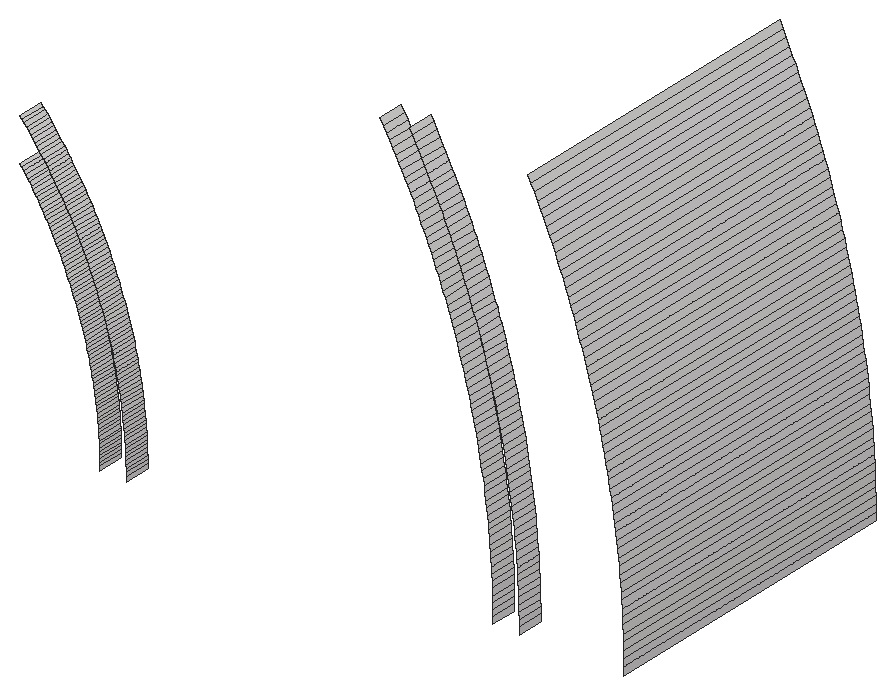
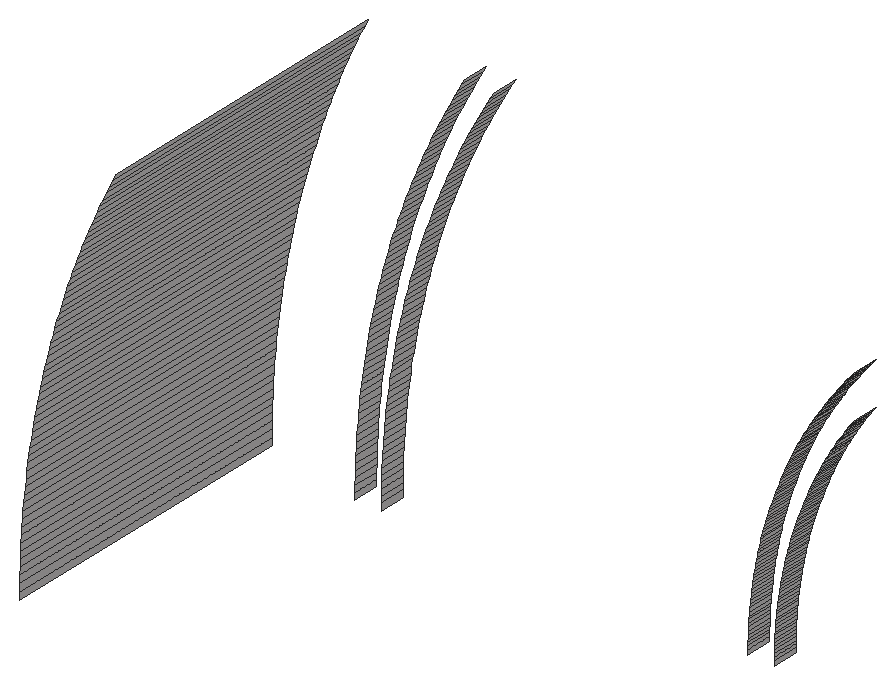
# SketchUp Ruby script. Lengths in inches.
U = 1.inch
M = Sketchup.active_model
def pt(a) = Geom::Point3d.new(a.map { |v| v * U })
def face(e, loops, mat)
  f = e.add_face(loops[0].map { |a| pt(a) })
  loops[1..].each { |l| e.add_face(l.map { |a| pt(a) }).erase! }
  f.material = f.back_material = mat if mat
  f
end
# faces: each face lists its corners as indices into pts; further lists are holes
def faces(e, pts, list, mat = nil) = list.each { |f| face(e, (f[0].is_a?(Array) ? f : [f]).map { |l| l.map { |i| pts[i] } }, mat) }
# xy, xz, yz: faces in a plane at the given z, y or x. An outline is a flat list of corners, or four numbers for a rectangle; further outlines are holes
def ring(l) = l.size == 4 ? [[l[0], l[1]], [l[2], l[1]], [l[2], l[3]], [l[0], l[3]]] : l.each_slice(2).to_a
def flat(e, list, mat, &to3) = list.each { |f| face(e, (f[0].is_a?(Array) ? f : [f]).map { |l| ring(l).map { |u, v| to3.(u, v) } }, mat) }
def xy(e, z, list, mat = nil) = flat(e, list, mat) { |x, y| [x, y, z] }
def xz(e, y, list, mat = nil) = flat(e, list, mat) { |x, z| [x, y, z] }
def yz(e, x, list, mat = nil) = flat(e, list, mat) { |y, z| [x, y, z] }
def lines(e, pts, list) = list.each { |a, b| e.add_line(pt(pts[a]), pt(pts[b])) }
# prism: a flat outline (further loops are holes) pulled along v
def prism(e, loops, v, mat = nil)
  f = face(e, loops, mat); d = Geom::Vector3d.new(v.map { |x| x * U })
  f.pushpull(f.normal.samedirection?(d) ? d.length : -d.length)
end
def box(e, o, s, mat = nil) = prism(e, [[o, [o[0] + s[0], o[1], o[2]], [o[0] + s[0], o[1] + s[1], o[2]], [o[0], o[1] + s[1], o[2]]]], [0, 0, s[2]], mat)
def at(x, y, z, deg = 0) = Geom::Transformation.translation(pt([x, y, z])) * Geom::Transformation.rotation(ORIGIN, Z_AXIS, deg.degrees)
def axes(o, x, y, z) = Geom::Transformation.new([*x, 0, *y, 0, *z, 0, *pt(o).to_a, 1])
def part(name) = M.definitions.add(name)
# library, detail: a bought-in or finely detailed component or shape, given as its bounding box
def library(name, o, s) = part(name).tap { |d| box(d.entities, o, s) }
def detail(e, o, s) = box(e.add_group.entities, o, s)
def put(e, d, t, mat = nil) = e.add_instance(d, t).tap { |i| i.material = mat if mat }
def group(e, t, mat = nil) = e.add_group.tap { |g| g.transformation = t; g.material = mat if mat }.entities
root = M.entities
M.materials.add("[Quartz Light Brown]").color = [215, 212, 212]
yz(root,519.98,[[38,84.75,39,84.88]],"[Quartz Light Brown]")
yz(root,519.99,[[38,84.5,39,84.63]],"[Quartz Light Brown]")
yz(root,520,[[38,83.96,39,84.125],[38,84.125,39,84.25],[38,84.25,39,84.375]],"[Quartz Light Brown]")
yz(root,520.97,[[38,84.93,39,85.07]],"[Quartz Light Brown]")
yz(root,520.99,[[38,84.53,39,84.67]],"[Quartz Light Brown]")
yz(root,521,[[38,83.96,39,84.13],[38,84.13,39,84.27],[38,84.27,39,84.4]],"[Quartz Light Brown]")
yz(root,534.98,[[38,84.97,39,85.22]],"[Quartz Light Brown]")
yz(root,535,[[38,83.99,39,84.24],[38,84.24,39,84.49]],"[Quartz Light Brown]")
yz(root,535.98,[[38,85.01,39,85.26]],"[Quartz Light Brown]")
yz(root,536,[[38,83.99,39,84.25],[38,84.25,39,84.5]],"[Quartz Light Brown]")
yz(root,540,[[38,84,50,84.28],[38,84.28,50,84.57]],"[Quartz Light Brown]")
p = [[519.99,39,84.5],[519.99,38,84.5],[520,38,84.375],[520,39,84.375],[520.99,38,84.53],[520.99,39,84.53],
  [521,39,84.4],[521,38,84.4],[534.99,39,84.73],[534.99,38,84.73],[535,38,84.49],[535,39,84.49],
  [535.99,38,84.75],[535.99,39,84.75],[536,39,84.5],[536,38,84.5],[519.98,39,84.75],[519.98,38,84.75],
  [519.99,38,84.63],[519.99,39,84.63],[539.99,38,84.85],[540,38,84.57],[540,50,84.57],[539.99,50,84.85],
  [520.98,38,84.8],[520.98,39,84.8],[520.99,39,84.67],[520.99,38,84.67],[534.98,39,84.97],[534.98,38,84.97],
  [520.97,38,84.93],[520.97,39,84.93],[535.98,38,85.01],[535.98,39,85.01],[539.98,38,85.13],[539.98,50,85.13],
  [519.97,39,85],[519.97,38,85],[519.98,38,84.88],[519.98,39,84.88],[519.96,39,85.13],[519.96,38,85.13],
  [519.95,39,85.26],[519.95,38,85.26],[520.96,38,85.2],[520.96,39,85.2],[520.97,39,85.07],[520.97,38,85.07],
  [539.97,38,85.41],[539.97,50,85.41],[520.95,38,85.33],[520.95,39,85.33],[534.97,39,85.46],[534.97,38,85.46],
  [534.98,38,85.22],[534.98,39,85.22],[519.94,39,85.38],[519.94,38,85.38],[520.9375,38,85.47],[520.9375,39,85.47],
  [535.96,38,85.51],[535.96,39,85.51],[535.98,39,85.26],[535.98,38,85.26],[519.93,39,85.51],[519.93,38,85.51],
  [539.96,38,85.7],[539.96,50,85.7],[519.92,39,85.63],[519.92,38,85.63],[520.92,38,85.6],[520.92,39,85.6],
  [534.95,39,85.7],[534.95,38,85.7],[535.95,38,85.76],[535.95,39,85.76],[519.9,39,85.76],[519.9,38,85.76],
  [520.91,38,85.73],[520.91,39,85.73],[520.9,38,85.87],[520.9,39,85.87],[534.9375,39,85.95],[534.9375,38,85.95],
  [539.95,38,85.98],[539.95,50,85.98],[519.89,39,85.88],[519.89,38,85.88],[535.9375,38,86.01],[535.9375,39,86.01],
  [519.875,39,86.01],[519.875,38,86.01],[520.88,38,86],[520.88,39,86],[534.92,39,86.1875],[534.92,38,86.1875],
  [519.86,39,86.13],[519.86,38,86.13],[520.87,38,86.13],[520.87,39,86.13],[535.92,38,86.26],[535.92,39,86.26],
  [539.93,38,86.26],[539.93,50,86.26],[519.84,39,86.25],[519.84,38,86.25],[520.85,38,86.26],[520.85,39,86.26],
  [534.9,39,86.43],[534.9,38,86.43],[519.82,39,86.38],[519.82,38,86.38],[520.83,38,86.4],[520.83,39,86.4],
  [535.9,38,86.51],[535.9,39,86.51],[539.91,38,86.54],[539.91,50,86.54],[519.8,39,86.5],[519.8,38,86.5],
  [520.8125,38,86.53],[520.8125,39,86.53],[534.88,39,86.67],[534.88,38,86.67],[519.78,39,86.625],[519.78,38,86.625],
  [520.79,38,86.66],[520.79,39,86.66],[535.88,38,86.76],[535.88,39,86.76],[539.89,38,86.82],[539.89,50,86.82],
  [519.76,39,86.75],[519.76,38,86.75],[520.77,38,86.79],[520.77,39,86.79],[534.86,39,86.92],[534.86,38,86.92],
  [519.74,39,86.875],[519.74,38,86.875],[520.75,38,86.92],[520.75,39,86.92],[535.86,38,87.01],[535.86,39,87.01],
  [539.87,38,87.11],[539.87,50,87.11],[519.72,39,87],[519.72,38,87],[520.72,38,87.05],[520.72,39,87.05],
  [534.84,39,87.16],[534.84,38,87.16],[519.69,39,87.12],[519.69,38,87.12],[535.83,38,87.26],[535.83,39,87.26],
  [519.67,39,87.24],[519.67,38,87.24],[520.7,38,87.19],[520.7,39,87.19],[539.84,38,87.39],[539.84,50,87.39],
  [519.64,39,87.37],[519.64,38,87.37],[520.67,38,87.32],[520.67,39,87.32],[534.8125,39,87.4],[534.8125,38,87.4],
  [520.65,38,87.45],[520.65,39,87.45],[535.81,38,87.51],[535.81,39,87.51],[519.61,39,87.49],[519.61,38,87.49],
  [520.62,38,87.58],[520.62,39,87.58],[534.79,39,87.64],[534.79,38,87.64],[539.8125,38,87.67],[539.8125,50,87.67],
  [519.59,39,87.61],[519.59,38,87.61],[535.78,38,87.76],[535.78,39,87.76],[519.56,39,87.74],[519.56,38,87.74],
  [520.59,38,87.71],[520.59,39,87.71],[534.76,39,87.89],[534.76,38,87.89],[519.53,39,87.86],[519.53,38,87.86],
  [520.5625,38,87.84],[520.5625,39,87.84],[539.78,38,87.95],[539.78,50,87.95],[520.53,38,87.97],[520.53,39,87.97],
  [535.75,38,88.01],[535.75,39,88.01],[519.5,39,87.98],[519.5,38,87.98],[534.72,39,88.125],[534.72,38,88.125],
  [519.47,39,88.1],[519.47,38,88.1],[520.5,38,88.1],[520.5,39,88.1],[535.72,38,88.26],[535.72,39,88.26],
  [539.75,38,88.23],[539.75,50,88.23],[519.43,39,88.22],[519.43,38,88.22],[520.47,38,88.23],[520.47,39,88.23],
  [534.69,39,88.37],[534.69,38,88.37],[519.4,39,88.34],[519.4,38,88.34],[520.43,38,88.36],[520.43,39,88.36],
  [539.72,38,88.51],[539.72,50,88.51],[519.36,39,88.46],[519.36,38,88.46],[535.68,38,88.51],[535.68,39,88.51],
  [520.4,38,88.49],[520.4,39,88.49],[534.66,39,88.61],[534.66,38,88.61],[519.33,39,88.58],[519.33,38,88.58],
  [520.36,38,88.61],[520.36,39,88.61],[535.64,38,88.76],[535.64,39,88.76],[539.68,38,88.79],[539.68,50,88.79],
  [519.29,39,88.7],[519.29,38,88.7],[520.32,38,88.74],[520.32,39,88.74],[534.62,39,88.85],[534.62,38,88.85],
  [519.26,39,88.82],[519.26,38,88.82],[520.29,38,88.87],[520.29,39,88.87],[519.22,39,88.94],[519.22,38,88.94],
  [534.58,39,89.09],[534.58,38,89.09],[535.61,38,89.01],[535.61,39,89.01],[539.64,38,89.07],[539.64,50,89.07],
  [519.18,39,89.0625],[519.18,38,89.0625],[520.25,38,89],[520.25,39,89],[520.21,38,89.125],[520.21,39,89.125],
  [535.57,38,89.25],[535.57,39,89.25],[519.14,39,89.18],[519.14,38,89.18],[520.17,38,89.25],[520.17,39,89.25],
  [534.54,39,89.33],[534.54,38,89.33],[539.6,38,89.35],[539.6,50,89.35],[519.1,39,89.3],[519.1,38,89.3],
  [519.05,39,89.42],[519.05,38,89.42],[520.125,38,89.38],[520.125,39,89.38],[534.5,39,89.57],[534.5,38,89.57],
  [535.52,38,89.5],[535.52,39,89.5],[519.01,39,89.54],[519.01,38,89.54],[520.08,38,89.51],[520.08,39,89.51],
  [539.56,38,89.63],[539.56,50,89.63],[518.97,39,89.66],[518.97,38,89.66],[520.04,38,89.63],[520.04,39,89.63],
  [535.48,38,89.75],[535.48,39,89.75],[519.99,38,89.76],[519.99,39,89.76],[534.45,39,89.81],[534.45,38,89.81],
  [539.51,38,89.91],[539.51,50,89.91],[518.92,39,89.77],[518.92,38,89.77],[535.43,38,90],[535.43,39,90],
  [518.875,39,89.89],[518.875,38,89.89],[519.95,38,89.88],[519.95,39,89.88],[534.4,39,90.05],[534.4,38,90.05],
  [518.83,39,90.01],[518.83,38,90.01],[519.9,38,90.01],[519.9,39,90.01],[539.46,38,90.1875],[539.46,50,90.1875],
  [518.78,39,90.12],[518.78,38,90.12],[519.85,38,90.13],[519.85,39,90.13],[534.36,39,90.29],[534.36,38,90.29],
  [535.39,38,90.24],[535.39,39,90.24],[518.73,39,90.24],[518.73,38,90.24],[519.81,38,90.26],[519.81,39,90.26],
  [518.68,39,90.35],[518.68,38,90.35],[535.34,38,90.49],[535.34,39,90.49],[539.41,38,90.47],[539.41,50,90.47],
  [519.76,38,90.38],[519.76,39,90.38],[534.31,39,90.52],[534.31,38,90.52],[518.63,39,90.47],[518.63,38,90.47],
  [519.71,38,90.51],[519.71,39,90.51],[518.58,39,90.58],[518.58,38,90.58],[519.65,38,90.63],[519.65,39,90.63],
  [534.25,39,90.76],[534.25,38,90.76],[535.28,38,90.74],[535.28,39,90.74],[539.36,38,90.75],[539.36,50,90.75],
  [518.53,39,90.7],[518.53,38,90.7],[519.6,38,90.75],[519.6,39,90.75],[518.48,39,90.8125],[518.48,38,90.8125],
  [535.23,38,90.98],[535.23,39,90.98],[539.31,38,91.02],[539.31,50,91.02],[518.42,39,90.93],[518.42,38,90.93],
  [519.55,38,90.875],[519.55,39,90.875],[534.2,39,91],[534.2,38,91],[518.37,39,91.04],[518.37,38,91.04],
  [519.49,38,91],[519.49,39,91],[518.3125,39,91.15],[518.3125,38,91.15],[519.4375,38,91.12],[519.4375,39,91.12],
  [534.14,39,91.24],[534.14,38,91.24],[535.17,38,91.23],[535.17,39,91.23],[539.25,38,91.3],[539.25,50,91.3],
  [519.38,38,91.24],[519.38,39,91.24],[518.26,39,91.26],[518.26,38,91.26],[519.32,38,91.36],[519.32,39,91.36],
  [534.09,39,91.47],[534.09,38,91.47],[535.12,38,91.47],[535.12,39,91.47],[518.2,39,91.375],[518.2,38,91.375],
  [539.19,38,91.58],[539.19,50,91.58],[518.14,39,91.49],[518.14,38,91.49],[519.27,38,91.48],[519.27,39,91.48],
  [518.08,39,91.6],[518.08,38,91.6],[519.21,38,91.6],[519.21,39,91.6],[534.03,39,91.71],[534.03,38,91.71],
  [535.06,38,91.71],[535.06,39,91.71],[518.02,39,91.71],[518.02,38,91.71],[519.15,38,91.72],[519.15,39,91.72],
  [539.13,38,91.85],[539.13,50,91.85],[517.96,39,91.82],[517.96,38,91.82],[519.09,38,91.84],[519.09,39,91.84],
  [533.96,39,91.94],[533.96,38,91.94],[534.99,38,91.96],[534.99,39,91.96],[517.9,39,91.93],[517.9,38,91.93],
  [519.02,38,91.95],[519.02,39,91.95],[517.84,39,92.04],[517.84,38,92.04],[533.9,39,92.18],[533.9,38,92.18],
  [539.07,38,92.13],[539.07,50,92.13],[517.77,39,92.14],[517.77,38,92.14],[518.96,38,92.07],[518.96,39,92.07],
  [534.93,38,92.2],[534.93,39,92.2],[517.71,39,92.25],[517.71,38,92.25],[518.9,38,92.19],[518.9,39,92.19],
  [539.01,38,92.4],[539.01,50,92.4],[518.83,38,92.31],[518.83,39,92.31],[533.84,39,92.41],[533.84,38,92.41],
  [534.87,38,92.44],[534.87,39,92.44],[517.64,39,92.36],[517.64,38,92.36],[518.77,38,92.42],[518.77,39,92.42],
  [517.58,39,92.47],[517.58,38,92.47],[518.7,38,92.54],[518.7,39,92.54],[533.77,39,92.65],[533.77,38,92.65],
  [534.8,38,92.6875],[534.8,39,92.6875],[538.9375,38,92.68],[538.9375,50,92.68],[517.51,39,92.57],[517.51,38,92.57],
  [518.63,38,92.65],[518.63,39,92.65],[517.44,39,92.68],[517.44,38,92.68],[533.7,39,92.88],[533.7,38,92.88],
  [517.37,39,92.78],[517.37,38,92.78],[518.5625,38,92.77],[518.5625,39,92.77],[534.73,38,92.93],[534.73,39,92.93],
  [538.87,38,92.95],[538.87,50,92.95],[517.3,39,92.89],[517.3,38,92.89],[518.49,38,92.88],[518.49,39,92.88],
  [517.23,39,92.99],[517.23,38,92.99],[518.42,38,93],[518.42,39,93],[533.63,39,93.12],[533.63,38,93.12],
  [534.66,38,93.17],[534.66,39,93.17],[517.16,39,93.1],[517.16,38,93.1],[518.35,38,93.11],[518.35,39,93.11],
  [538.8,38,93.23],[538.8,50,93.23],[517.09,39,93.2],[517.09,38,93.2],[518.28,38,93.22],[518.28,39,93.22],
  [533.56,39,93.35],[533.56,38,93.35],[517.02,39,93.3],[517.02,38,93.3],[518.21,38,93.33],[518.21,39,93.33],
  [534.59,38,93.41],[534.59,39,93.41],[538.72,38,93.5],[538.72,50,93.5],[516.94,39,93.4],[516.94,38,93.4],
  [518.13,38,93.44],[518.13,39,93.44],[533.48,39,93.58],[533.48,38,93.58],[518.06,38,93.56],[518.06,39,93.56],
  [534.51,38,93.65],[534.51,39,93.65],[538.65,38,93.77],[538.65,50,93.77],[517.98,38,93.67],[517.98,39,93.67],
  [533.41,39,93.8125],[533.41,38,93.8125],[534.43,38,93.89],[534.43,39,93.89],[517.91,38,93.78],[517.91,39,93.78],
  [517.83,38,93.88],[517.83,39,93.88],[533.33,39,94.04],[533.33,38,94.04],[538.57,38,94.04],[538.57,50,94.04],
  [517.75,38,93.99],[517.75,39,93.99],[534.36,38,94.13],[534.36,39,94.13],[517.67,38,94.1],[517.67,39,94.1],
  [533.25,39,94.27],[533.25,38,94.27],[538.49,38,94.31],[538.49,50,94.31],[517.59,38,94.21],[517.59,39,94.21],
  [534.27,38,94.37],[534.27,39,94.37],[517.51,38,94.3125],[517.51,39,94.3125],[517.43,38,94.42],[517.43,39,94.42],
  [533.17,39,94.5],[533.17,38,94.5],[538.41,38,94.59],[538.41,50,94.59],[517.35,38,94.52],[517.35,39,94.52],
  [534.19,38,94.6],[534.19,39,94.6],[517.27,38,94.63],[517.27,39,94.63],[533.08,39,94.73],[533.08,38,94.73],
  [517.18,38,94.73],[517.18,39,94.73],[534.11,38,94.84],[534.11,39,94.84],[538.32,38,94.86],[538.32,50,94.86],
  [517.1,38,94.84],[517.1,39,94.84],[533,39,94.96],[533,38,94.96],[517.01,38,94.9375],[517.01,39,94.9375],
  [534.02,38,95.08],[534.02,39,95.08],[516.93,38,95.04],[516.93,39,95.04],[538.24,38,95.125],[538.24,50,95.125],
  [532.91,39,95.19],[532.91,38,95.19],[533.93,38,95.3125],[533.93,39,95.3125],[538.15,38,95.39],[538.15,50,95.39],
  [532.82,39,95.41],[532.82,38,95.41],[533.84,38,95.55],[533.84,39,95.55],[532.73,39,95.64],[532.73,38,95.64],
  [538.06,38,95.66],[538.06,50,95.66],[533.75,38,95.78],[533.75,39,95.78],[532.64,39,95.86],[532.64,38,95.86],
  [537.97,38,95.93],[537.97,50,95.93],[533.66,38,96.01],[533.66,39,96.01],[532.55,39,96.09],[532.55,38,96.09],
  [537.87,38,96.19],[537.87,50,96.19],[533.5625,38,96.25],[533.5625,39,96.25],[532.45,39,96.3125],[532.45,38,96.3125],
  [533.47,38,96.48],[533.47,39,96.48],[537.77,38,96.46],[537.77,50,96.46],[532.35,39,96.53],[532.35,38,96.53],
  [532.25,39,96.76],[532.25,38,96.76],[533.37,38,96.71],[533.37,39,96.71],[537.68,38,96.73],[537.68,50,96.73],
  [533.27,38,96.9375],[533.27,39,96.9375],[537.58,38,96.99],[537.58,50,96.99],[532.15,39,96.98],[532.15,38,96.98],
  [533.16,38,97.17],[533.16,39,97.17],[532.05,39,97.2],[532.05,38,97.2],[537.47,38,97.25],[537.47,50,97.25],
  [531.95,39,97.42],[531.95,38,97.42],[533.0625,38,97.4],[533.0625,39,97.4],[537.37,38,97.51],[537.37,50,97.51],
  [531.84,39,97.64],[531.84,38,97.64],[532.95,38,97.625],[532.95,39,97.625],[537.26,38,97.78],[537.26,50,97.78],
  [531.73,39,97.86],[531.73,38,97.86],[532.85,38,97.85],[532.85,39,97.85],[537.15,38,98.04],[537.15,50,98.04],
  [531.62,39,98.07],[531.62,38,98.07],[532.74,38,98.08],[532.74,39,98.08],[537.04,38,98.3],[537.04,50,98.3],
  [531.51,39,98.29],[531.51,38,98.29],[532.625,38,98.3],[532.625,39,98.3],[531.4,39,98.51],[531.4,38,98.51],
  [532.51,38,98.53],[532.51,39,98.53],[536.93,38,98.56],[536.93,50,98.56],[531.28,39,98.72],[531.28,38,98.72],
  [532.4,38,98.75],[532.4,39,98.75],[536.8125,38,98.81],[536.8125,50,98.81],[531.17,39,98.93],[531.17,38,98.93],
  [532.28,38,98.97],[532.28,39,98.97],[536.69,38,99.07],[536.69,50,99.07],[531.05,39,99.15],[531.05,38,99.15],
  [532.16,38,99.2],[532.16,39,99.2],[530.93,39,99.36],[530.93,38,99.36],[536.57,38,99.33],[536.57,50,99.33],
  [532.04,38,99.42],[532.04,39,99.42],[536.45,38,99.58],[536.45,50,99.58],[530.81,39,99.57],[530.81,38,99.57],
  [531.92,38,99.64],[531.92,39,99.64],[530.68,39,99.78],[530.68,38,99.78],[531.8,38,99.85],[531.8,39,99.85],
  [536.33,38,99.84],[536.33,50,99.84]]
faces(root,p,[[0,1,2,3],[4,5,6,7],[8,9,10,11],[12,13,14,15],[16,17,18,19],[20,21,22,23],[24,25,26,27],[28,29,9,8],
  [30,31,25,24],[32,33,13,12],[34,20,23,35],[36,37,38,39],[40,41,37,36],[42,43,41,40],[44,45,46,47],[48,34,35,49],
  [50,51,45,44],[52,53,54,55],[56,57,43,42],[58,59,51,50],[60,61,62,63],[64,65,57,56],[66,48,49,67],[68,69,65,64],
  [70,71,59,58],[72,73,53,52],[74,75,61,60],[76,77,69,68],[78,79,71,70],[80,81,79,78],[82,83,73,72],[84,66,67,85],
  [86,87,77,76],[88,89,75,74],[90,91,87,86],[92,93,81,80],[94,95,83,82],[96,97,91,90],[98,99,93,92],[100,101,89,88],
  [102,84,85,103],[104,105,97,96],[106,107,99,98],[108,109,95,94],[110,111,105,104],[112,113,107,106],[114,115,101,100],[116,102,103,117],
  [118,119,111,110],[120,121,113,112],[122,123,109,108],[124,125,119,118],[126,127,121,120],[128,129,115,114],[130,116,117,131],[132,133,125,124],
  [134,135,127,126],[136,137,123,122],[138,139,133,132],[140,141,135,134],[142,143,129,128],[144,130,131,145],[146,147,139,138],[148,149,141,140],
  [150,151,137,136],[152,153,147,146],[154,155,143,142],[156,157,153,152],[158,159,149,148],[160,144,145,161],[162,163,157,156],[164,165,159,158],
  [166,167,151,150],[168,169,165,164],[170,171,155,154],[172,173,163,162],[174,175,169,168],[176,177,167,166],[178,160,161,179],[180,181,173,172],
  [182,183,171,170],[184,185,181,180],[186,187,175,174],[188,189,177,176],[190,191,185,184],[192,193,187,186],[194,178,179,195],[196,197,193,192],
  [198,199,183,182],[200,201,191,190],[202,203,189,188],[204,205,201,200],[206,207,197,196],[208,209,199,198],[210,194,195,211],[212,213,205,204],
  [214,215,207,206],[216,217,203,202],[218,219,213,212],[220,221,215,214],[222,210,211,223],[224,225,219,218],[226,227,209,208],[228,229,221,220],
  [230,231,217,216],[232,233,225,224],[234,235,229,228],[236,237,227,226],[238,222,223,239],[240,241,233,232],[242,243,235,234],[244,245,231,230],
  [246,247,241,240],[248,249,243,242],[250,251,247,246],[252,253,245,244],[254,255,237,236],[256,238,239,257],[258,259,251,250],[260,261,249,248],
  [262,263,261,260],[264,265,255,254],[266,267,259,258],[268,269,263,262],[270,271,253,252],[272,256,257,273],[274,275,267,266],[276,277,275,274],
  [278,279,269,268],[280,281,271,270],[282,283,265,264],[284,285,277,276],[286,287,279,278],[288,272,273,289],[290,291,285,284],[292,293,287,286],
  [294,295,283,282],[296,297,293,292],[298,299,281,280],[300,288,289,301],[302,303,291,290],[304,305,295,294],[306,307,303,302],[308,309,297,296],
  [310,311,299,298],[312,313,307,306],[314,315,309,308],[316,300,301,317],[318,319,313,312],[320,321,315,314],[322,323,311,310],[324,325,305,304],
  [326,327,319,318],[328,329,321,320],[330,331,327,326],[332,333,325,324],[334,316,317,335],[336,337,329,328],[338,339,323,322],[340,341,331,330],
  [342,343,337,336],[344,345,341,340],[346,347,343,342],[348,349,339,338],[350,351,333,332],[352,334,335,353],[354,355,345,344],[356,357,347,346],
  [358,359,355,354],[360,361,351,350],[362,352,353,363],[364,365,359,358],[366,367,357,356],[368,369,349,348],[370,371,365,364],[372,373,367,366],
  [374,375,371,370],[376,377,373,372],[378,379,369,368],[380,381,361,360],[382,362,363,383],[384,385,377,376],[386,387,375,374],[388,389,385,384],
  [390,391,379,378],[392,393,381,380],[394,395,387,386],[396,382,383,397],[398,399,395,394],[400,401,389,388],[402,403,399,398],[404,405,401,400],
  [406,407,391,390],[408,409,393,392],[410,411,403,402],[412,413,405,404],[414,396,397,415],[416,417,411,410],[418,419,413,412],[420,421,407,406],
  [422,423,409,408],[424,425,417,416],[426,427,419,418],[428,429,425,424],[430,431,421,420],[432,414,415,433],[434,435,429,428],[436,437,427,426],
  [438,439,423,422],[440,441,435,434],[442,443,437,436],[444,432,433,445],[446,447,443,442],[448,449,431,430],[450,451,439,438],[452,453,441,440],
  [454,455,447,446],[456,457,453,452],[458,459,455,454],[460,461,449,448],[462,463,451,450],[464,444,445,465],[466,467,457,456],[468,469,459,458],
  [470,471,467,466],[472,473,461,460],[474,475,471,470],[476,477,469,468],[478,479,463,462],[480,464,465,481],[482,483,475,474],[484,485,477,476],
  [486,487,483,482],[488,489,485,484],[490,491,473,472],[492,493,479,478],[494,495,487,486],[496,497,489,488],[498,480,481,499],[500,501,495,494],
  [502,503,497,496],[504,505,491,490],[506,507,501,500],[508,509,503,502],[510,511,493,492],[512,498,499,513],[514,515,507,506],[516,517,509,508],
  [518,519,505,504],[520,521,517,516],[522,523,511,510],[524,512,513,525],[526,527,521,520],[528,529,519,518],[530,531,523,522],[532,533,527,526],
  [534,535,533,532],[536,537,529,528],[538,524,525,539],[540,541,535,534],[542,543,531,530],[544,545,541,540],[546,547,537,536],[548,538,539,549],
  [550,551,545,544],[552,553,543,542],[554,555,551,550],[556,557,555,554],[558,559,547,546],[560,548,549,561],[562,563,557,556],[564,565,553,552],
  [566,567,563,562],[568,569,559,558],[570,571,567,566],[572,573,565,564],[574,560,561,575],[576,577,571,570],[578,579,569,568],[580,581,577,576],
  [582,583,573,572],[584,585,581,580],[586,574,575,587],[588,589,579,578],[590,591,583,582],[592,586,587,593],[594,595,589,588],[596,597,591,590],
  [598,599,595,594],[600,592,593,601],[602,603,597,596],[604,605,599,598],[606,600,601,607],[608,609,603,602],[610,611,605,604],[612,606,607,613],
  [614,615,609,608],[616,617,611,610],[618,619,615,614],[620,612,613,621],[622,623,617,616],[624,625,623,622],[626,627,619,618],[628,620,621,629],
  [630,631,627,626],[632,628,629,633],[634,635,625,624],[636,637,631,630],[638,639,635,634],[640,632,633,641],[642,643,639,638],[644,645,637,636],
  [646,640,641,647],[648,649,643,642],[650,651,645,644],[652,646,647,653],[654,655,649,648],[656,657,651,650],[658,652,653,659],[660,661,655,654],
  [662,663,657,656],[664,658,659,665],[666,667,661,660],[668,669,663,662],[670,671,667,666],[672,673,669,668],[674,664,665,675],[676,677,671,670],
  [678,679,673,672],[680,674,675,681],[682,683,677,676],[684,685,679,678],[686,680,681,687],[688,689,683,682],[690,691,685,684],[692,693,689,688],
  [694,686,687,695],[696,697,691,690],[698,694,695,699],[700,701,693,692],[702,703,697,696],[704,705,701,700],[706,707,703,702],[708,698,699,709]],"[Quartz Light Brown]")
